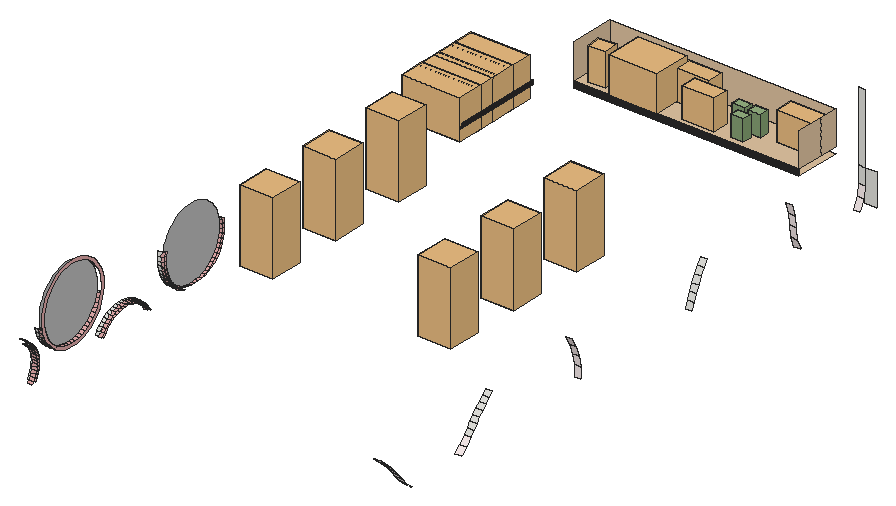
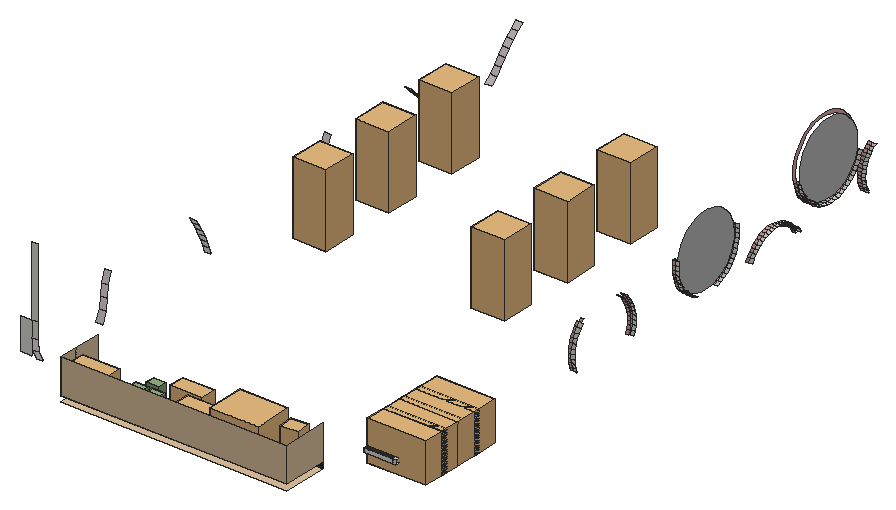
# SketchUp Ruby script. Lengths in inches.
U = 1.inch
M = Sketchup.active_model
def pt(a) = Geom::Point3d.new(a.map { |v| v * U })
def face(e, loops, mat)
  f = e.add_face(loops[0].map { |a| pt(a) })
  loops[1..].each { |l| e.add_face(l.map { |a| pt(a) }).erase! }
  f.material = f.back_material = mat if mat
  f
end
# faces: each face lists its corners as indices into pts; further lists are holes
def faces(e, pts, list, mat = nil) = list.each { |f| face(e, (f[0].is_a?(Array) ? f : [f]).map { |l| l.map { |i| pts[i] } }, mat) }
# xy, xz, yz: faces in a plane at the given z, y or x. An outline is a flat list of corners, or four numbers for a rectangle; further outlines are holes
def ring(l) = l.size == 4 ? [[l[0], l[1]], [l[2], l[1]], [l[2], l[3]], [l[0], l[3]]] : l.each_slice(2).to_a
def flat(e, list, mat, &to3) = list.each { |f| face(e, (f[0].is_a?(Array) ? f : [f]).map { |l| ring(l).map { |u, v| to3.(u, v) } }, mat) }
def xy(e, z, list, mat = nil) = flat(e, list, mat) { |x, y| [x, y, z] }
def xz(e, y, list, mat = nil) = flat(e, list, mat) { |x, z| [x, y, z] }
def yz(e, x, list, mat = nil) = flat(e, list, mat) { |y, z| [x, y, z] }
def lines(e, pts, list) = list.each { |a, b| e.add_line(pt(pts[a]), pt(pts[b])) }
# prism: a flat outline (further loops are holes) pulled along v
def prism(e, loops, v, mat = nil)
  f = face(e, loops, mat); d = Geom::Vector3d.new(v.map { |x| x * U })
  f.pushpull(f.normal.samedirection?(d) ? d.length : -d.length)
end
def box(e, o, s, mat = nil) = prism(e, [[o, [o[0] + s[0], o[1], o[2]], [o[0] + s[0], o[1] + s[1], o[2]], [o[0], o[1] + s[1], o[2]]]], [0, 0, s[2]], mat)
def at(x, y, z, deg = 0) = Geom::Transformation.translation(pt([x, y, z])) * Geom::Transformation.rotation(ORIGIN, Z_AXIS, deg.degrees)
def axes(o, x, y, z) = Geom::Transformation.new([*x, 0, *y, 0, *z, 0, *pt(o).to_a, 1])
def part(name) = M.definitions.add(name)
# library, detail: a bought-in or finely detailed component or shape, given as its bounding box
def library(name, o, s) = part(name).tap { |d| box(d.entities, o, s) }
def detail(e, o, s) = box(e.add_group.entities, o, s)
def put(e, d, t, mat = nil) = e.add_instance(d, t).tap { |i| i.material = mat if mat }
def group(e, t, mat = nil) = e.add_group.tap { |g| g.transformation = t; g.material = mat if mat }.entities
root = M.entities
M.materials.add("Generic").color = [224, 169, 169]
M.materials.add("Generic\#1").color = [44, 42, 42]
M.materials.add("Generic\#2").color = [246, 234, 234]
M.materials.add("Generic\#3").color = [224, 196, 161]
M.materials.add("QQ截图20130319210408\#1").color = [134, 161, 117]
M.materials.add("QQ截图20130319210422\#1").color = [134, 163, 115]
M.materials.add("QQ截图20130319210439\#1").color = [149, 178, 130]
M.materials.add("[Mirror 01]").color = [185, 185, 185]
c1 = library("Untitled (6)",[-101.41,0,-4.6],[35.6,35.6,49.16])
c2 = library("Group\#668",[-1.42,-1.42,0],[20.03,45.75,30.81])
c3 = part("组\#1")
xy(c3.entities,0,[[0,0,4.33,3.15]],"QQ截图20130319210439\#1")
xy(c3.entities,7.09,[[0,0,4.33,3.15]],"QQ截图20130319210439\#1")
xz(c3.entities,0,[[0,0,4.33,7.09]],"QQ截图20130319210408\#1")
xz(c3.entities,3.15,[[0,0,4.33,7.09]],"QQ截图20130319210408\#1")
yz(c3.entities,0,[[0,0,3.15,7.09]],"QQ截图20130319210422\#1")
yz(c3.entities,4.33,[[0,0,3.15,7.09]],"QQ截图20130319210422\#1")
c4 = part("无标题")
put(c4.entities,c3,at(0,0,0))
c5 = library("Group\#667",[0,0,0],[8.32,16.8,15.65])
c6 = library("Demitasse-2",[1.91,3.34,-0.76],[4.02,5.2,11.56])
c7 = library("Group\#637",[-1.61,-1.61,0],[18.66,14.41,13.77])
c8 = library("Group\#638",[0,0,0],[22.58,10.85,16.9375])
xy(root,68.36,[[34.93,453.375,150.42,476.6875]],"Generic\#3")
xy(root,71.49,[[34.875,453.375,150.375,476.6875]],"Generic\#3")
xy(root,72.8125,[[9,393.02,10.6875,439.14]])
xy(root,72.8125,[[10.6875,393.02,25.625,439.14]],"Generic\#1")
xy(root,75,[[9,393.02,10.6875,439.14]])
xy(root,75,[[10.6875,393.02,25.625,439.14]],"Generic\#1")
xz(root,393.02,[[9,72.8125,10.6875,75]])
xz(root,393.02,[[10.6875,72.8125,25.625,75]],"Generic\#1")
xz(root,439.14,[[9,72.8125,10.6875,75],[10.6875,72.8125,25.625,75]])
xz(root,453.375,[[184.0625,67.8125,190,84.1],[180.9375,75.96,184.0625,84.1],[180.9375,84.1,184.0625,120]])
xz(root,453.375,[[34.93,68.36,150.42,68.36,150.375,71.49,34.875,71.49]],"Generic\#1")
xz(root,476.6875,[[34.875,71.49,150.375,89.18]],"Generic\#3")
yz(root,10.6875,[[239.5625,64.78,241.62,64.98,243.65,65.4,245.61,66.06,247.49,66.93,249.25,68.01,250.88,69.29,252.35,70.75,253.65,72.36,254.75,74.11,255.65,75.97,256.33,77.93,256.78,79.95,257,82,256.99,84.07,256.74,86.13,256.25,88.14,255.54,90.08,254.61,91.93,253.48,93.66,252.16,95.26,250.66,96.6875,249.01,97.9375,247.23,98.99,245.34,99.84,243.37,100.46,241.34,100.86,239.28,101.02,237.21,100.94,235.16,100.63,233.16,100.09,231.24,99.32,229.42,98.34,227.72,97.16,226.17,95.79,224.78,94.26,223.58,92.57,222.57,90.76,221.78,88.85,221.22,86.86,220.88,84.82,220.78,82.75,220.91,80.6875,221.28,78.65,221.88,76.67,222.7,74.77,223.73,72.98,224.96,71.3125,226.37,69.8,227.95,68.45,229.66,67.3,231.5,66.35,233.4375,65.61,235.44,65.1,237.49,64.82],[160.47,72.17,162.58,72.3125,164.65,72.7,166.66,73.3125,168.59,74.15,170.41,75.21,172.1,76.47,173.64,77.91,175,79.52,176.17,81.27,177.13,83.14,177.87,85.12,178.39,87.16,178.66,89.25,178.7,91.35,178.49,93.45,178.05,95.51,177.38,97.5,176.48,99.41,175.375,101.2,174.07,102.85,172.58,104.35,170.9375,105.66,169.15,106.78,167.25,107.69,165.26,108.375,163.2,108.83,161.11,109.05,159,109.02,156.91,108.76,154.87,108.26,152.89,107.53,151.01,106.58,149.25,105.42,147.64,104.07,146.1875,102.54,144.92,100.86,143.85,99.04,143,97.11,142.37,95.1,141.98,93.03,141.82,90.93,141.9,88.83,142.23,86.75,142.79,84.72,143.57,82.76,144.58,80.91,145.78,79.1875,147.18,77.61,148.75,76.2,150.47,74.99,152.3125,73.97,154.26,73.17,156.29,72.6,158.37,72.27]],"[Mirror 01]")
yz(root,13,[[[160.49,70.77,162.75,70.92,164.98,71.34,167.15,72,169.22,72.9,171.18,74.04,173,75.39,174.65,76.95,176.12,78.68,177.38,80.56,178.41,82.58,179.21,84.7,179.76,86.9,180.06,89.14,180.1,91.41,179.88,93.66,179.4,95.88,178.68,98.03,177.71,100.08,176.52,102.01,175.12,103.78,173.52,105.39,171.75,106.81,169.83,108.01,167.78,108.99,165.64,109.72,163.43,110.21,161.17,110.44,158.91,110.42,156.66,110.14,154.46,109.6,152.33,108.8125,150.31,107.79,148.42,106.54,146.68,105.09,145.12,103.44,143.75,101.63,142.61,99.68,141.6875,97.61,141.01,95.44,140.59,93.22,140.42,90.96,140.51,88.69,140.86,86.45,141.46,84.27,142.3,82.17,143.38,80.17,144.68,78.32,146.1875,76.62,147.875,75.11,149.72,73.8,151.71,72.71,153.81,71.85,155.99,71.23,158.23,70.87],[160.47,72.17,158.37,72.27,156.29,72.6,154.26,73.17,152.3125,73.97,150.47,74.99,148.75,76.2,147.18,77.61,145.78,79.1875,144.58,80.91,143.57,82.76,142.79,84.72,142.23,86.75,141.9,88.83,141.82,90.93,141.98,93.03,142.37,95.1,143,97.11,143.85,99.04,144.92,100.86,146.1875,102.54,147.64,104.07,149.25,105.42,151.01,106.58,152.89,107.53,154.87,108.26,156.91,108.76,159,109.02,161.11,109.05,163.2,108.83,165.26,108.375,167.25,107.69,169.15,106.78,170.9375,105.66,172.58,104.35,174.07,102.85,175.375,101.2,176.48,99.41,177.38,97.5,178.05,95.51,178.49,93.45,178.7,91.35,178.66,89.25,178.39,87.16,177.87,85.12,177.13,83.14,176.17,81.27,175,79.52,173.64,77.91,172.1,76.47,170.41,75.21,168.59,74.15,166.66,73.3125,164.65,72.7,162.58,72.3125]]],"Generic")
yz(root,25.625,[[393.02,72.8125,439.14,75]],"Generic\#1")
yz(root,34.875,[[453.375,71.49,476.6875,89.18]],"Generic\#3")
yz(root,150.375,[[453.375,71.49,467.1875,89.18],[467.1875,71.49,476.6875,89.18]],"Generic\#3")
p = [[10.6875,135.33,65.55],[10.6875,134.44,64.33],[12.9375,134.44,64.33],[12.9375,135.33,65.55],[10.6875,323.43,64.36],[10.6875,324.17,66.48],
  [9,324.17,66.48],[9,323.43,64.36],[12,324.17,66.48],[12,323.43,64.36],[10.6875,231.01,65.24],[10.6875,233.07,64.45],
  [9,233.07,64.45],[9,231.01,65.24],[12.1875,233.07,64.45],[12.1875,231.01,65.24],[10.6875,136.54,64.77],[10.6875,137.36,66.23],
  [9,137.36,66.23],[9,136.54,64.77],[12.9375,137.36,66.23],[12.9375,136.54,64.77],[10.6875,210.93,64.82],[10.6875,209.95,66.58],
  [9,209.95,66.58],[9,210.93,64.82],[12.375,209.95,66.58],[12.375,210.93,64.82],[10.6875,237.49,64.82],[10.6875,235.44,65.1],
  [12.1875,235.44,65.1],[12.1875,237.49,64.82],[10.6875,239.5625,64.78],[12.1875,239.5625,64.78],[10.6875,241.62,64.98],[12.1875,241.62,64.98],
  [10.6875,246.06,64.93],[10.6875,248.0625,65.86],[9,248.0625,65.86],[9,246.06,64.93],[12.1875,248.0625,65.86],[12.1875,246.06,64.93],
  [10.6875,322.7,66.9],[10.6875,322.02,64.94],[12,322.02,64.94],[12,322.7,66.9],[184.0625,412.21,64.92],[184.0625,410,70.25],
  [180.9375,410,70.25],[180.9375,412.21,64.92],[184.0625,452.625,70.25],[184.0625,450.42,64.92],[180.9375,450.42,64.92],[180.9375,452.625,70.25],
  [10.6875,243.65,65.4],[12.1875,243.65,65.4],[10.6875,233.4375,65.61],[12.1875,233.4375,65.61],[10.6875,286.17,67.26],[10.6875,286.82,65.12],
  [9,286.82,65.12],[9,286.17,67.26],[12,286.82,65.12],[12,286.17,67.26],[184.0625,163.1875,65.17],[184.0625,159.9375,67.94],
  [180.9375,159.9375,67.94],[180.9375,163.1875,65.17],[184.0625,198.44,67.94],[184.0625,195.19,65.17],[180.9375,195.19,65.17],[180.9375,198.44,67.94],
  [10.6875,229.05,66.25],[9,229.05,66.25],[12.1875,229.05,66.25],[10.6875,180.97,65.27],[10.6875,181.98,66.83],[12.375,181.98,66.83],
  [12.375,180.97,65.27],[10.6875,245.61,66.06],[12.1875,245.61,66.06],[10.6875,136.0625,66.87],[12.9375,136.0625,66.87],[10.6875,231.5,66.35],
  [12.1875,231.5,66.35],[10.6875,288.25,65.64],[10.6875,287.65,67.62],[12,287.65,67.62],[12,288.25,65.64],[10.6875,180.98,67.57],
  [10.6875,179.89,65.89],[9,179.89,65.89],[9,180.98,67.57],[12.375,179.89,65.89],[12.375,180.98,67.57],[10.6875,207.8125,67.42],
  [10.6875,208.9,65.91],[12.375,208.9,65.91],[12.375,207.8125,67.42],[10.6875,249.94,67.02],[9,249.94,67.02],[12.1875,249.94,67.02],
  [10.6875,247.49,66.93],[12.1875,247.49,66.93],[10.6875,138.01,67.77],[9,138.01,67.77],[12.9375,138.01,67.77],[10.6875,227.21,67.49],
  [9,227.21,67.49],[12.1875,227.21,67.49],[10.6875,229.66,67.3],[12.1875,229.66,67.3],[10.6875,324.66,68.67],[9,324.66,68.67],
  [12,324.66,68.67],[10.6875,208.78,68.2],[9,208.78,68.2],[12.375,208.78,68.2],[10.6875,183.17,68.27],[12.375,183.17,68.27],
  [10.6875,136.65,68.25],[12.9375,136.65,68.25],[10.6875,249.25,68.01],[12.1875,249.25,68.01],[10.6875,323.15,68.92],[12,323.15,68.92],
  [184.0625,343.94,70.36],[184.0625,342.6875,66.9375],[180.9375,342.6875,66.9375],[180.9375,343.94,70.36],[10.6875,251.68,68.38],[9,251.68,68.38],
  [12.1875,251.68,68.38],[184.0625,271.43,67.11],[184.0625,271.55,72.61],[180.9375,271.55,72.61],[180.9375,271.43,67.11],[10.6875,227.95,68.45],
  [12.1875,227.95,68.45],[10.6875,285.77,69.47],[9,285.77,69.47],[12,285.77,69.47],[10.6875,206.5625,68.8],[12.375,206.5625,68.8],
  [10.6875,225.53,68.92],[9,225.53,68.92],[12.1875,225.53,68.92],[10.6875,182.26,69.11],[9,182.26,69.11],[12.375,182.26,69.11],
  [10.6875,287.28,69.66],[12,287.28,69.66],[10.6875,138.48,69.375],[9,138.48,69.375],[12.9375,138.48,69.375],[184.0625,157.16,71.1875],
  [180.9375,157.16,71.1875],[184.0625,201.22,71.1875],[180.9375,201.22,71.1875],[10.6875,250.88,69.29],[12.1875,250.88,69.29],[10.6875,207.4375,69.69],
  [9,207.4375,69.69],[12.375,207.4375,69.69],[10.6875,137.07,69.7],[12.9375,137.07,69.7],[10.6875,184.52,69.56],[12.375,184.52,69.56],
  [10.6875,253.25,69.93],[9,253.25,69.93],[12.1875,253.25,69.93],[10.6875,226.37,69.8],[12.1875,226.37,69.8],[10.6875,324.89,70.9],
  [9,324.89,70.9],[12,324.89,70.9],[10.6875,205.16,70.03],[12.375,205.16,70.03],[10.6875,224.03,70.53],[9,224.03,70.53],
  [12.1875,224.03,70.53],[10.6875,323.375,70.97],[12,323.375,70.97],[10.6875,183.7,70.5],[9,183.7,70.5],[12.375,183.7,70.5],
  [10.6875,252.35,70.75],[12.1875,252.35,70.75],[10.6875,138.76,71.02],[9,138.76,71.02],[12.9375,138.76,71.02],[10.6875,285.625,71.71],
  [9,285.625,71.71],[12,285.625,71.71],[10.6875,186,70.69],[12.375,186,70.69],[10.6875,137.32,71.18],[12.9375,137.32,71.18],
  [10.6875,205.93,71.01],[9,205.93,71.01],[12.375,205.93,71.01],[10.6875,287.15,71.72],[12,287.15,71.72],[10.6875,224.96,71.3125],
  [12.1875,224.96,71.3125],[10.6875,254.64,71.65],[9,254.64,71.65],[12.1875,254.64,71.65],[10.6875,203.63,71.09],[12.375,203.63,71.09],
  [184.0625,409.25,75.96],[180.9375,409.25,75.96],[184.0625,453.375,75.96],[180.9375,453.375,75.96],[184.0625,345.35,73.73],[180.9375,345.35,73.73],
  [10.6875,185.3,71.72],[9,185.3,71.72],[12.375,185.3,71.72],[10.6875,222.71,72.3125],[9,222.71,72.3125],[12.1875,222.71,72.3125],
  [10.6875,187.6,71.64],[12.375,187.6,71.64],[10.6875,253.65,72.36],[12.1875,253.65,72.36],[10.6875,158.23,70.87],[10.6875,160.49,70.77],
  [9,160.49,70.77],[9,158.23,70.87],[13,160.49,70.77],[13,158.23,70.87],[10.6875,162.75,70.92],[9,162.75,70.92],
  [13,162.75,70.92],[10.6875,155.99,71.23],[9,155.99,71.23],[13,155.99,71.23],[10.6875,164.98,71.34],[9,164.98,71.34],
  [13,164.98,71.34],[10.6875,324.875,73.14],[9,324.875,73.14],[12,324.875,73.14],[10.6875,138.85,72.69],[9,138.85,72.69],
  [12.9375,138.85,72.69],[10.6875,204.28,72.15],[9,204.28,72.15],[12.375,204.28,72.15],[10.6875,323.36,73.04],[12,323.36,73.04],
  [10.6875,201.99,71.97],[12.375,201.99,71.97],[10.6875,137.41,72.6875],[12.9375,137.41,72.6875],[10.6875,153.81,71.85],[9,153.81,71.85],
  [13,153.81,71.85],[184.0625,154.72,74.36],[180.9375,154.72,74.36],[184.0625,202.98,73.52],[180.9375,202.98,73.52],[10.6875,167.15,72],
  [9,167.15,72],[13,167.15,72],[10.6875,223.73,72.98],[12.1875,223.73,72.98],[10.6875,189.3,72.4],[12.375,189.3,72.4],
  [10.6875,187.02,72.74],[9,187.02,72.74],[12.375,187.02,72.74],[10.6875,255.82,73.52],[9,255.82,73.52],[12.1875,255.82,73.52],
  [10.6875,285.73,73.95],[9,285.73,73.95],[12,285.73,73.95],[10.6875,287.25,73.79],[12,287.25,73.79],[10.6875,151.71,72.71],
  [9,151.71,72.71],[13,151.71,72.71],[10.6875,169.22,72.9],[9,169.22,72.9],[13,169.22,72.9],[10.6875,200.26,72.65],
  [12.375,200.26,72.65],[10.6875,160.47,72.17],[10.6875,158.37,72.27],[13,158.37,72.27],[13,160.47,72.17],[10.6875,162.58,72.3125],
  [13,162.58,72.3125],[10.6875,202.51,73.1],[9,202.51,73.1],[12.375,202.51,73.1],[10.6875,156.29,72.6],[13,156.29,72.6],
  [10.6875,164.65,72.7],[13,164.65,72.7],[10.6875,221.61,74.22],[9,221.61,74.22],[12.1875,221.61,74.22],[10.6875,191.07,72.97],
  [12.375,191.07,72.97],[10.6875,254.75,74.11],[12.1875,254.75,74.11],[10.6875,154.26,73.17],[13,154.26,73.17],[184.0625,270.64,78.03],
  [180.9375,270.64,78.03],[10.6875,137.32,74.19],[12.9375,137.32,74.19],[10.6875,138.75,74.36],[9,138.75,74.36],[12.9375,138.75,74.36],
  [10.6875,149.72,73.8],[9,149.72,73.8],[13,149.72,73.8],[10.6875,166.66,73.3125],[13,166.66,73.3125],[10.6875,188.85,73.57],
  [9,188.85,73.57],[12.375,188.85,73.57],[10.6875,198.46,73.14],[12.375,198.46,73.14],[10.6875,171.18,74.04],[9,171.18,74.04],
  [13,171.18,74.04],[10.6875,192.9,73.33],[12.375,192.9,73.33],[10.6875,222.7,74.77],[12.1875,222.7,74.77],[10.6875,323.11,75.1],
  [12,323.11,75.1],[10.6875,196.62,73.41],[12.375,196.62,73.41],[10.6875,200.65,73.84],[9,200.65,73.84],[12.375,200.65,73.84],
  [10.6875,324.6,75.37],[9,324.6,75.37],[12,324.6,75.37],[10.6875,152.3125,73.97],[13,152.3125,73.97],[10.6875,168.59,74.15],
  [13,168.59,74.15],[10.6875,194.75,73.48],[12.375,194.75,73.48],[184.0625,204.8,75.8],[180.9375,204.8,75.8],[10.6875,256.77,75.51],
  [9,256.77,75.51],[12.1875,256.77,75.51],[10.6875,190.76,74.18],[9,190.76,74.18],[12.375,190.76,74.18],[184.0625,346.9,77.02],
  [180.9375,346.9,77.02],[10.6875,147.875,75.11],[9,147.875,75.11],[13,147.875,75.11],[10.6875,198.71,74.36],[9,198.71,74.36],
  [12.375,198.71,74.36],[10.6875,287.58,75.83],[12,287.58,75.83],[10.6875,150.47,74.99],[13,150.47,74.99],[10.6875,173,75.39],
  [9,173,75.39],[13,173,75.39],[10.6875,286.1,76.16],[9,286.1,76.16],[12,286.1,76.16],[10.6875,255.65,75.97],
  [12.1875,255.65,75.97],[10.6875,137.06,75.67],[12.9375,137.06,75.67],[10.6875,170.41,75.21],[13,170.41,75.21],[10.6875,192.73,74.5625],
  [9,192.73,74.5625],[12.375,192.73,74.5625],[10.6875,220.74,76.25],[9,220.74,76.25],[12.1875,220.74,76.25],[10.6875,138.47,76],
  [9,138.47,76],[12.9375,138.47,76],[184.0625,152.1,77.39],[180.9375,152.1,77.39],[10.6875,196.73,74.65],[9,196.73,74.65],
  [12.375,196.73,74.65],[10.6875,194.73,74.72],[9,194.73,74.72],[12.375,194.73,74.72],[10.6875,221.88,76.67],[12.1875,221.88,76.67],
  [10.6875,148.75,76.2],[13,148.75,76.2],[10.6875,146.1875,76.62],[9,146.1875,76.62],[13,146.1875,76.62],[10.6875,322.62,77.11],
  [12,322.62,77.11],[10.6875,172.1,76.47],[13,172.1,76.47],[10.6875,174.65,76.95],[9,174.65,76.95],[13,174.65,76.95],
  [10.6875,324.08,77.55],[9,324.08,77.55],[12,324.08,77.55],[10.6875,257.5,77.59],[9,257.5,77.59],[12.1875,257.5,77.59],
  [10.6875,136.63,77.12],[12.9375,136.63,77.12],[184.0625,206.7,78.01],[180.9375,206.7,78.01],[10.6875,288.15,77.82],[12,288.15,77.82],
  [10.6875,137.99,77.61],[9,137.99,77.61],[12.9375,137.99,77.61],[10.6875,256.33,77.93],[12.1875,256.33,77.93],[184.0625,408.67,81.6875],
  [180.9375,408.67,81.6875],[10.6875,147.18,77.61],[13,147.18,77.61],[10.6875,286.71,78.32],[9,286.71,78.32],[12,286.71,78.32],
  [10.6875,220.1,78.37],[9,220.1,78.37],[12.1875,220.1,78.37],[10.6875,173.64,77.91],[13,173.64,77.91],[10.6875,144.68,78.32],
  [9,144.68,78.32],[13,144.68,78.32],[10.6875,221.28,78.65],[12.1875,221.28,78.65],[10.6875,176.12,78.68],[9,176.12,78.68],
  [13,176.12,78.68],[184.0625,348.6,80.25],[180.9375,348.6,80.25],[10.6875,136.04,78.5],[12.9375,136.04,78.5],[10.6875,321.91,79.05],
  [12,321.91,79.05],[184.0625,149.34,80.28],[180.9375,149.34,80.28],[10.6875,137.34,79.14],[9,137.34,79.14],[12.9375,137.34,79.14],
  [10.6875,145.78,79.1875],[13,145.78,79.1875],[10.6875,257.98,79.75],[9,257.98,79.75],[12.1875,257.98,79.75],[10.6875,323.31,79.66],
  [9,323.31,79.66],[12,323.31,79.66],[10.6875,288.94,79.73],[12,288.94,79.73],[10.6875,175,79.52],[13,175,79.52],
  [10.6875,256.78,79.95],[12.1875,256.78,79.95],[184.0625,208.66,80.17],[180.9375,208.66,80.17],[184.0625,268.73,83.18],[180.9375,268.73,83.18],
  [10.6875,143.38,80.17],[9,143.38,80.17],[13,143.38,80.17],[10.6875,287.57,80.39],[9,287.57,80.39],[12,287.57,80.39],
  [10.6875,219.71,80.54],[9,219.71,80.54],[12.1875,219.71,80.54],[10.6875,135.3,79.8125],[12.9375,135.3,79.8125],[10.6875,177.38,80.56],
  [9,177.38,80.56],[13,177.38,80.56],[10.6875,220.91,80.6875],[12.1875,220.91,80.6875],[10.6875,136.52,80.6],[9,136.52,80.6],
  [12.9375,136.52,80.6],[10.6875,320.98,80.9],[12,320.98,80.9],[10.6875,144.58,80.91],[13,144.58,80.91],[10.6875,176.17,81.27],
  [13,176.17,81.27],[10.6875,258.22,81.94],[9,258.22,81.94],[12.1875,258.22,81.94],[10.6875,289.95,81.54],[12,289.95,81.54],
  [10.6875,322.3,81.66],[9,322.3,81.66],[12,322.3,81.66],[10.6875,134.41,81.03],[12.9375,134.41,81.03],[10.6875,257,82],
  [12.1875,257,82],[10.6875,142.3,82.17],[9,142.3,82.17],[13,142.3,82.17],[184.0625,210.68,82.27],[180.9375,210.68,82.27],
  [184.0625,146.41,83.01],[180.9375,146.41,83.01],[184.0625,350.45,83.4],[180.9375,350.45,83.4],[10.6875,288.66,82.36],[9,288.66,82.36],
  [12,288.66,82.36],[10.6875,219.5625,82.74],[9,219.5625,82.74],[12.1875,219.5625,82.74],[10.6875,135.53,81.95],[9,135.53,81.95],
  [12.9375,135.53,81.95],[10.6875,178.41,82.58],[9,178.41,82.58],[13,178.41,82.58],[10.6875,220.78,82.75],[12.1875,220.78,82.75],
  [10.6875,143.57,82.76],[13,143.57,82.76],[10.6875,319.85,82.64],[12,319.85,82.64],[10.6875,133.39,82.14],[12.9375,133.39,82.14],
  [10.6875,177.13,83.14],[13,177.13,83.14],[10.6875,291.15,83.23],[12,291.15,83.23],[10.6875,321.07,83.54],[9,321.07,83.54],
  [12,321.07,83.54],[184.0625,406.96,87.1875],[180.9375,406.96,87.1875],[10.6875,134.4,83.18],[9,134.4,83.18],[12.9375,134.4,83.18],
  [10.6875,258.2,84.15],[9,258.2,84.15],[12.1875,258.2,84.15],[10.6875,256.99,84.07],[12.1875,256.99,84.07],[10.6875,132.25,83.12],
  [12.9375,132.25,83.12],[10.6875,141.46,84.27],[9,141.46,84.27],[13,141.46,84.27],[184.0625,212.78,84.31],[180.9375,212.78,84.31],
  [10.6875,289.96,84.18],[9,289.96,84.18],[12,289.96,84.18],[10.6875,179.21,84.7],[9,179.21,84.7],[13,179.21,84.7],
  [10.6875,318.53,84.23],[12,318.53,84.23],[10.6875,219.67,84.95],[9,219.67,84.95],[12.1875,219.67,84.95],[10.6875,142.79,84.72],
  [13,142.79,84.72],[10.6875,220.88,84.82],[12.1875,220.88,84.82],[184.0625,143.35,85.58],[180.9375,143.35,85.58],[10.6875,131.01,83.97],
  [12.9375,131.01,83.97],[10.6875,177.87,85.12],[13,177.87,85.12],[10.6875,133.14,84.27],[9,133.14,84.27],[12.9375,133.14,84.27],
  [184.0625,265.88,87.89],[180.9375,265.88,87.89],[10.6875,292.54,84.76],[12,292.54,84.76],[184.0625,352.42,86.46],[180.9375,352.42,86.46],
  [10.6875,319.64,85.27],[9,319.64,85.27],[12,319.64,85.27],[10.6875,256.74,86.13],[12.1875,256.74,86.13],[10.6875,257.93,86.34],
  [9,257.93,86.34],[12.1875,257.93,86.34],[10.6875,291.47,85.85],[9,291.47,85.85],[12,291.47,85.85],[10.6875,317.03,85.66],
  [12,317.03,85.66],[10.6875,131.75,85.21],[9,131.75,85.21],[12.9375,131.75,85.21],[10.6875,140.86,86.45],[9,140.86,86.45],
  [13,140.86,86.45],[184.0625,214.93,86.28],[180.9375,214.93,86.28],[10.6875,142.23,86.75],[13,142.23,86.75],[10.6875,179.76,86.9],
  [9,179.76,86.9],[13,179.76,86.9],[10.6875,221.22,86.86],[12.1875,221.22,86.86],[10.6875,294.09,86.13],[12,294.09,86.13],
  [10.6875,220.03,87.125],[9,220.03,87.125],[12.1875,220.03,87.125],[10.6875,178.39,87.16],[13,178.39,87.16]]
faces(root,p,[[0,1,2,3],[4,5,8,9],[10,11,14,15],[16,17,20,21],[22,23,26,27],[28,29,30,31],[32,28,31,33],[34,32,33,35],
  [36,37,40,41],[42,43,44,45],[54,34,35,55],[29,56,57,30],[58,59,62,63],[72,10,15,74],[75,76,77,78],[79,54,55,80],
  [81,0,3,82],[56,83,84,57],[85,86,87,88],[89,90,93,94],[95,96,97,98],[37,99,101,40],[102,79,80,103],[17,104,106,20],
  [107,72,74,109],[83,110,111,84],[5,112,114,8],[23,115,117,26],[76,118,119,77],[120,81,82,121],[122,102,103,123],[124,42,45,125],
  [99,130,132,101],[110,137,138,111],[139,58,63,141],[142,95,98,143],[144,107,109,146],[147,89,94,149],[86,150,151,87],[104,152,154,106],
  [159,122,123,160],[115,161,163,117],[164,120,121,165],[118,166,167,119],[130,168,170,132],[137,171,172,138],[112,173,175,114],[176,142,143,177],
  [178,144,146,180],[181,124,125,182],[183,147,149,185],[186,159,160,187],[152,188,190,154],[191,139,141,193],[166,194,195,167],[196,164,165,197],
  [161,198,200,163],[150,201,202,151],[171,203,204,172],[168,205,207,170],[208,176,177,209],[216,183,185,218],[219,178,180,221],[194,222,223,195],
  [224,186,187,225],[226,227,230,231],[227,232,234,230],[235,226,231,237],[232,238,240,234],[173,241,243,175],[188,244,246,190],[198,247,249,200],
  [250,181,182,251],[252,208,209,253],[254,196,197,255],[256,235,237,258],[238,263,265,240],[203,266,267,204],[222,268,269,223],[270,216,218,272],
  [205,273,275,207],[276,191,193,278],[201,279,280,202],[281,256,258,283],[263,284,286,265],[287,252,253,288],[289,290,291,292],[293,289,292,294],
  [247,295,297,249],[290,298,299,291],[300,293,294,301],[302,219,221,304],[268,305,306,269],[307,224,225,308],[298,309,310,299],[313,254,255,314],
  [244,315,317,246],[318,281,283,320],[321,300,301,322],[323,270,272,325],[326,287,288,327],[284,328,330,286],[305,331,332,306],[266,333,334,267],
  [335,250,251,336],[337,326,327,338],[295,339,341,297],[241,342,344,243],[309,345,346,310],[347,321,322,348],[331,349,350,332],[349,337,338,350],
  [273,353,355,275],[356,323,325,358],[361,318,320,363],[339,364,366,341],[279,367,368,280],[345,369,370,346],[328,371,373,330],[374,276,278,376],
  [377,307,308,378],[379,313,314,380],[381,347,348,382],[383,356,358,385],[386,302,304,388],[315,389,391,317],[364,394,396,366],[397,383,385,399],
  [394,397,399,396],[333,400,401,334],[369,402,403,370],[404,361,363,406],[407,335,336,408],[409,381,382,410],[371,411,413,373],[342,414,416,344],
  [353,417,419,355],[420,379,380,421],[367,424,425,368],[389,426,428,391],[429,377,378,430],[402,433,434,403],[435,374,376,437],[438,386,388,440],
  [441,409,410,442],[443,404,406,445],[400,446,447,401],[411,448,450,413],[453,420,421,454],[455,407,408,456],[426,459,461,428],[433,462,463,434],
  [417,464,466,419],[414,467,469,416],[424,470,471,425],[472,441,442,473],[474,429,430,475],[480,443,445,482],[483,435,437,485],[486,438,440,488],
  [489,453,454,490],[448,491,493,450],[446,494,495,447],[459,496,498,461],[499,455,456,500],[462,501,502,463],[503,472,473,504],[464,505,507,466],
  [470,508,509,471],[467,510,512,469],[513,489,490,514],[515,474,475,516],[517,480,482,519],[526,483,485,528],[529,486,488,531],[496,532,534,498],
  [491,535,537,493],[494,538,539,495],[501,540,541,502],[542,499,500,543],[544,513,514,545],[546,503,504,547],[508,548,549,509],[510,550,552,512],
  [532,555,557,534],[505,558,560,507],[561,515,516,562],[563,544,545,564],[565,517,519,567],[570,526,528,572],[535,573,575,537],[576,542,543,577],
  [578,529,531,580],[540,581,582,541],[538,583,584,539],[587,563,564,588],[589,546,547,590],[555,591,593,557],[548,596,597,549],[550,600,602,552],
  [603,561,562,604],[558,605,607,560],[608,570,572,610],[611,576,577,612],[591,613,615,593],[616,565,567,618],[581,621,622,582],[573,623,625,575],
  [583,626,627,584],[596,628,629,597],[630,578,580,632],[633,589,590,634]],"Generic")
faces(root,p,[[4,5,6,7],[10,11,12,13],[16,17,18,19],[22,23,24,25],[36,37,38,39],[58,59,60,61],[72,10,13,73],[89,90,91,92],
  [37,99,100,38],[17,104,105,18],[107,72,73,108],[5,112,113,6],[23,115,116,24],[126,127,128,129],[99,130,131,100],[139,58,61,140],
  [144,107,108,145],[147,89,92,148],[104,152,153,105],[115,161,162,116],[130,168,169,131],[112,173,174,113],[178,144,145,179],[183,147,148,184],
  [152,188,189,153],[191,139,140,192],[161,198,199,162],[168,205,206,169],[214,126,129,215],[216,183,184,217],[219,178,179,220],[226,227,228,229],
  [227,232,233,228],[235,226,229,236],[232,238,239,233],[173,241,242,174],[188,244,245,189],[198,247,248,199],[256,235,236,257],[261,157,158,262],
  [238,263,264,239],[270,216,217,271],[205,273,274,206],[276,191,192,277],[281,256,257,282],[263,284,285,264],[247,295,296,248],[302,219,220,303],
  [244,315,316,245],[318,281,282,319],[323,270,271,324],[284,328,329,285],[295,339,340,296],[241,342,343,242],[351,261,262,352],[273,353,354,274],
  [356,323,324,357],[359,214,215,360],[361,318,319,362],[339,364,365,340],[328,371,372,329],[374,276,277,375],[383,356,357,384],[386,302,303,387],
  [315,389,390,316],[364,394,395,365],[397,383,384,398],[394,397,398,395],[404,361,362,405],[371,411,412,372],[342,414,415,343],[353,417,418,354],
  [422,351,352,423],[389,426,427,390],[435,374,375,436],[438,386,387,439],[443,404,405,444],[411,448,449,412],[451,359,360,452],[426,459,460,427],
  [417,464,465,418],[414,467,468,415],[476,422,423,477],[480,443,444,481],[483,435,436,484],[486,438,439,487],[448,491,492,449],[459,496,497,460],
  [464,505,506,465],[467,510,511,468],[517,480,481,518],[520,476,477,521],[524,451,452,525],[526,483,484,527],[529,486,487,530],[496,532,533,497],
  [491,535,536,492],[510,550,551,511],[532,555,556,533],[505,558,559,506],[565,517,518,566],[568,520,521,569],[570,526,527,571],[535,573,574,536],
  [578,529,530,579],[555,591,592,556],[598,524,525,599],[550,600,601,551],[558,605,606,559],[608,570,571,609],[591,613,614,592],[616,565,566,617],
  [619,568,569,620],[573,623,624,574],[630,578,579,631]])
faces(root,p,[[46,47,48,49],[50,51,52,53],[64,65,66,67],[68,69,70,71],[133,134,135,136],[65,155,156,66],[157,68,71,158],[47,210,211,48],
  [212,50,53,213],[155,259,260,156],[134,311,312,135],[259,392,393,260],[210,431,432,211],[392,457,458,393],[311,478,479,312],[457,522,523,458],
  [431,553,554,432],[522,585,586,523],[478,594,595,479]],"Generic\#2")
put(root,c1,axes([86.15,236.48,86.14],[0.48,0,0],[0,0.48,0],[0,0,0.7584]))
put(root,c1,axes([177.4,236.48,86.14],[0.48,0,0],[0,0.48,0],[0,0,0.7584]))
put(root,c1,axes([86.15,276.8,86.14],[0.48,0,0],[0,0.48,0],[0,0,0.7584]))
put(root,c1,axes([177.4,276.8,86.14],[0.48,0,0],[0,0.48,0],[0,0,0.7584]))
put(root,c1,axes([86.15,317.11,86.14],[0.48,0,0],[0,0.48,0],[0,0,0.7584]))
put(root,c1,axes([177.4,317.11,86.14],[0.48,0,0],[0,0.48,0],[0,0,0.7584]))
put(root,c2,axes([24.6875,393.47,67.14],[0,0.6557,0],[-0.6557,0,0],[0,0,0.6557]))
put(root,c2,axes([24.6875,403.85,67.14],[0,0.6557,0],[-0.6557,0,0],[0,0,0.6557]))
put(root,c2,axes([24.6875,414.22,67.14],[0,0.6557,0],[-0.6557,0,0],[0,0,0.6557]))
put(root,c2,axes([24.6875,424.6,67.14],[0,0.6557,0],[-0.6557,0,0],[0,0,0.6557]))
put(root,c4,axes([112.55,456.8125,71.49],[1.4915,0,0],[0,1.4915,0],[0,0,1.4915]))
put(root,c5,axes([88.18,464.3,71.49],[0,-0.98136,0],[0.98136,0,0],[0,0,0.98136]))
put(root,c6,axes([33.45,466.7,72.59],[0.17709,-1.85774,0],[1.67197,0.15938,0],[0,0,1.43551]))
put(root,c7,axes([54.92,455.51,71.49],[1.329,0,0],[0,1.329,0],[0,0,1.329]))
put(root,c4,axes([107.47,464.03,71.49],[1.4915,0,0],[0,1.4915,0],[0,0,1.4915]))
put(root,c4,axes([115.85,464.03,71.49],[1.4915,0,0],[0,1.4915,0],[0,0,1.4915]))
put(root,c5,axes([77.55,474.16,71.49],[0,-0.98136,0],[0.98136,0,0],[0,0,0.98136]))
put(root,c8,axes([129.17,465.4375,71.49],[0.85882,0,0],[0,0.85882,0],[0,0,0.85882]))
